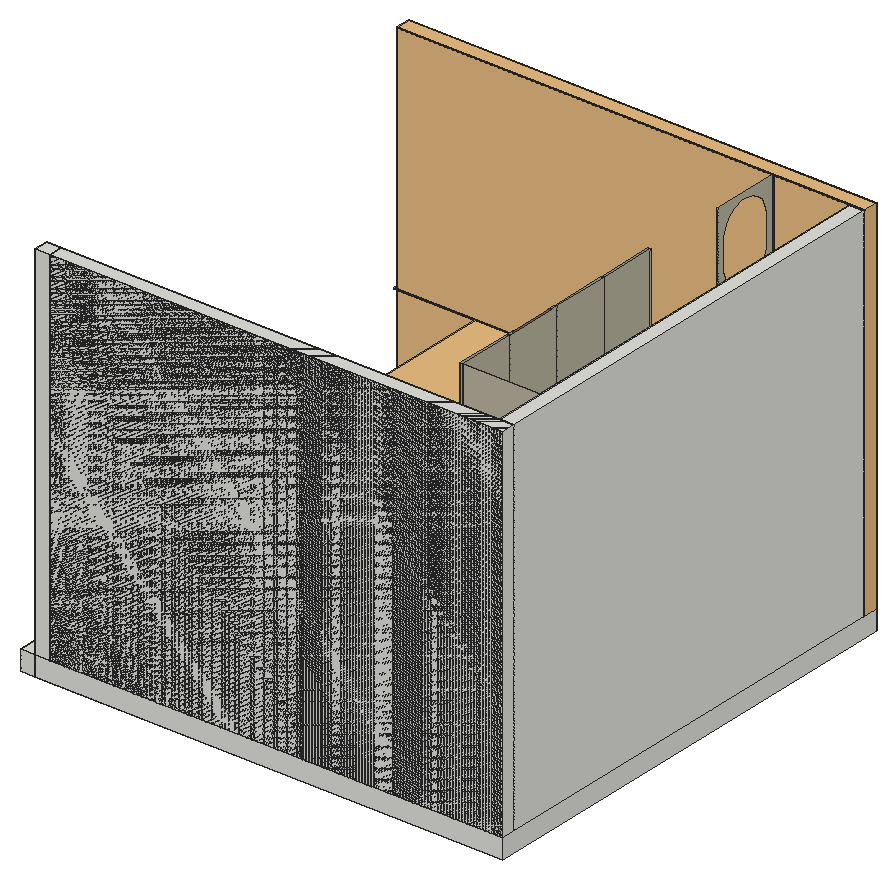
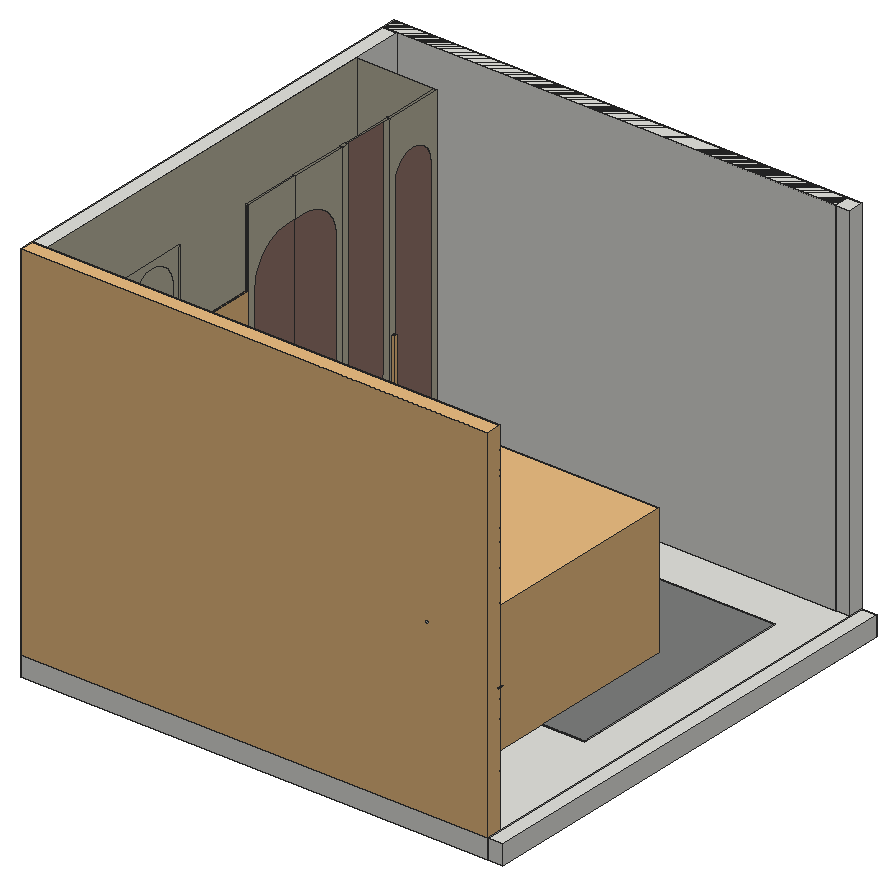
# SketchUp Ruby script. Lengths in inches.
U = 1.inch
M = Sketchup.active_model
def pt(a) = Geom::Point3d.new(a.map { |v| v * U })
def face(e, loops, mat)
  f = e.add_face(loops[0].map { |a| pt(a) })
  loops[1..].each { |l| e.add_face(l.map { |a| pt(a) }).erase! }
  f.material = f.back_material = mat if mat
  f
end
# faces: each face lists its corners as indices into pts; further lists are holes
def faces(e, pts, list, mat = nil) = list.each { |f| face(e, (f[0].is_a?(Array) ? f : [f]).map { |l| l.map { |i| pts[i] } }, mat) }
# xy, xz, yz: faces in a plane at the given z, y or x. An outline is a flat list of corners, or four numbers for a rectangle; further outlines are holes
def ring(l) = l.size == 4 ? [[l[0], l[1]], [l[2], l[1]], [l[2], l[3]], [l[0], l[3]]] : l.each_slice(2).to_a
def flat(e, list, mat, &to3) = list.each { |f| face(e, (f[0].is_a?(Array) ? f : [f]).map { |l| ring(l).map { |u, v| to3.(u, v) } }, mat) }
def xy(e, z, list, mat = nil) = flat(e, list, mat) { |x, y| [x, y, z] }
def xz(e, y, list, mat = nil) = flat(e, list, mat) { |x, z| [x, y, z] }
def yz(e, x, list, mat = nil) = flat(e, list, mat) { |y, z| [x, y, z] }
def lines(e, pts, list) = list.each { |a, b| e.add_line(pt(pts[a]), pt(pts[b])) }
# prism: a flat outline (further loops are holes) pulled along v
def prism(e, loops, v, mat = nil)
  f = face(e, loops, mat); d = Geom::Vector3d.new(v.map { |x| x * U })
  f.pushpull(f.normal.samedirection?(d) ? d.length : -d.length)
end
def box(e, o, s, mat = nil) = prism(e, [[o, [o[0] + s[0], o[1], o[2]], [o[0] + s[0], o[1] + s[1], o[2]], [o[0], o[1] + s[1], o[2]]]], [0, 0, s[2]], mat)
def at(x, y, z, deg = 0) = Geom::Transformation.translation(pt([x, y, z])) * Geom::Transformation.rotation(ORIGIN, Z_AXIS, deg.degrees)
def axes(o, x, y, z) = Geom::Transformation.new([*x, 0, *y, 0, *z, 0, *pt(o).to_a, 1])
def part(name) = M.definitions.add(name)
# library, detail: a bought-in or finely detailed component or shape, given as its bounding box
def library(name, o, s) = part(name).tap { |d| box(d.entities, o, s) }
def detail(e, o, s) = box(e.add_group.entities, o, s)
def put(e, d, t, mat = nil) = e.add_instance(d, t).tap { |i| i.material = mat if mat }
def group(e, t, mat = nil) = e.add_group.tap { |g| g.transformation = t; g.material = mat if mat }.entities
root = M.entities
M.materials.add("DDR840RVS01100X").color = [126, 127, 125]
M.materials.add("Olon-Blank-Canvas-VF300-1K").color = [237, 238, 234]
M.materials.add("Tafisa-Terrarossa-PM780-4K").color = [148, 117, 107]
M.materials.add("Uniboard-L19-Putty-4K").color = [187, 181, 160]
c1 = library("Group\#10",[-0.5,-0.5,-0.1],[116.2,1.51,0.2])
c2 = library("Group149\#1",[-72,-56,0],[144,112,0.24])
c3 = part("Carpet v15 (4)")
xy(c3.entities,0,[[-70.87,0,47.24,78.74]])
xy(c3.entities,0.39,[[-70.87,0,47.24,78.74]],"DDR840RVS01100X")
xz(c3.entities,0,[[-70.87,0,47.24,0.39]])
xz(c3.entities,78.74,[[-70.87,0,47.24,0.39]])
yz(c3.entities,-70.87,[[0,0,78.74,0.39]])
yz(c3.entities,47.24,[[0,0,78.74,0.39]])
c4 = library("Crowd Pleaser Bed",[-34.48,-45.67,0],[68.96,91.51,40.05])
c5 = library("Group39\#2",[-12.88,-41.94,0],[25.76,83.88,0.5])
c6 = library("Block 237 020",[-7.27,-8.35,0],[14.55,16.7,1.34])
c7 = part("Component\#11")
detail(c7.entities,[0,0,0],[0.1875,0.74,16.72])
c8 = library("Group\#26",[-0.5,-0.5,0],[2,18,8.5])
c9 = library("Cabinet knob",[0,0,0],[1.34,1.34,0.92])
c10 = library("Group\#23",[-0.5,-0.5,-0.1],[2,18,0.2])
c11 = library("Interior Props 221 030",[-2.57,-3.63,-0.04],[5.13,7.27,11.89])
c12 = library("Group\#24",[-0.5,-0.5,0],[2,18,8.5])
c13 = library("Candle 296 011",[-2.88,-2.88,-0.03],[5.76,5.76,9.25])
c14 = library("Group\#22",[-0.5,-0.5,-0.1],[2,18,0.2])
c15 = library("Interior Props 221 025",[-7.35,-1.5,-10.4],[14.7,1.56,20.81])
c16 = library("Group\#21",[-0.5,-0.5,-0.1],[2,18,0.2])
c17 = library("Decorative Deer 209 004",[-1.58,-4.16,0],[3.36,7.25,10.63])
xy(root,6,[[122,20.22,144,139.5]],"Uniboard-L19-Putty-4K")
xy(root,10,[[119.29,56.62,119.29,58.62,119.53,58.62,119.53,74.5,120,74.5,120,56.62],[119.53,74.62,119.53,90.5,119.29,90.5,119.29,92.5,120,92.5,120,74.62]],"Tafisa-Terrarossa-PM780-4K")
xy(root,10,[[119.29,20.22,119.29,22.22,119.53,22.22,119.53,36.36,119.29,36.36,119.29,38.24,120,38.24,120,20.22],[120,20.22,122,51.5],[119.29,38.36,120,51.5],[119.29,51.5,120,56.5],[120,51.5,120,92.5,122,87.5,122,51.5],
  [122,87.5,120,92.5,120,118.5,122,123.5],[119.96,92.62,120,118.38],[120,118.5,120,139.38,120.71,139.38,120.71,139.5,122,139.5,122,123.5]],"Uniboard-L19-Putty-4K")
xy(root,17.69,[[119.29,38.36,120,56.5]],"Uniboard-L19-Putty-4K")
xy(root,17.8125,[[119.29,38.36,120,56.5]],"Uniboard-L19-Putty-4K")
xy(root,23.65,[[120,120.5,141.83,137.5]],"Uniboard-L19-Putty-4K")
xy(root,24.35,[[120,120.5,142.83,137.5]],"Uniboard-L19-Putty-4K")
xy(root,25.51,[[119.29,38.36,120,56.5]],"Uniboard-L19-Putty-4K")
xy(root,25.625,[[119.29,38.36,120,56.5]],"Uniboard-L19-Putty-4K")
xy(root,33.32,[[119.29,38.36,120,56.5]],"Uniboard-L19-Putty-4K")
xy(root,33.4375,[[119.29,38.36,120,56.5]],"Uniboard-L19-Putty-4K")
xy(root,41.13,[[119.29,38.36,120,56.5]],"Uniboard-L19-Putty-4K")
xy(root,41.25,[[119.29,38.36,120,56.5]],"Uniboard-L19-Putty-4K")
xy(root,46.5,[[120,120.5,141.83,137.5]],"Uniboard-L19-Putty-4K")
xy(root,47.21,[[120,120.5,142.83,137.5]],"Uniboard-L19-Putty-4K")
xy(root,63.29,[[120,120.5,141.83,137.5]],"Uniboard-L19-Putty-4K")
xy(root,64,[[120,120.5,142.83,137.5]],"Uniboard-L19-Putty-4K")
xz(root,20.22,[[122,6,144,6,144,118,120,118,120,10,122,10],[119.29,10,120,117.88]],"Uniboard-L19-Putty-4K")
xz(root,22.22,[[119.29,10,119.53,99.06]],"Tafisa-Terrarossa-PM780-4K")
xz(root,36.36,[[119.29,10,119.53,99.06]],"Tafisa-Terrarossa-PM780-4K")
xz(root,38.24,[[119.29,10,120,117.88]],"Uniboard-L19-Putty-4K")
xz(root,38.36,[[119.29,10,120,17.69],[119.29,17.8125,120,25.51],[119.29,25.51,120,25.625],[119.29,25.625,120,33.32],[119.29,33.4375,120,41.13],
  [119.29,41.25,120,117.88]],"Uniboard-L19-Putty-4K")
xz(root,40.36,[[119.29,50.32,119.53,117.88]],"Tafisa-Terrarossa-PM780-4K")
xz(root,54.5,[[119.29,50.32,119.53,117.88]],"Tafisa-Terrarossa-PM780-4K")
xz(root,56.5,[[119.29,10,120,17.69],[119.29,17.8125,120,25.51],[119.29,25.625,120,33.32],[119.29,33.4375,120,41.13],[119.29,41.25,119.29,117.88,119.53,117.88,119.53,118,120,118,120,41.25]],"Uniboard-L19-Putty-4K")
xz(root,56.62,[[119.29,10,120,117.88]],"Uniboard-L19-Putty-4K")
xz(root,58.62,[[119.29,10,119.53,94.14]],"Tafisa-Terrarossa-PM780-4K")
xz(root,74.5,[[119.53,10,119.53,106.125,119.29,106.125,119.29,117.88,120,117.88,120,10]],"Tafisa-Terrarossa-PM780-4K")
xz(root,74.62,[[119.53,10,120,10,120,117.88,119.29,117.88,119.29,106.125,119.53,106.125]],"Tafisa-Terrarossa-PM780-4K")
xz(root,90.5,[[119.29,10,119.53,93.8125]],"Tafisa-Terrarossa-PM780-4K")
xz(root,92.5,[[119.29,10,120,117.88]],"Uniboard-L19-Putty-4K")
xz(root,92.62,[[119.96,10,120,93.88]],"Uniboard-L19-Putty-4K")
xz(root,118.38,[[119.96,10,120,93.88]],"Uniboard-L19-Putty-4K")
xz(root,120.5,[[120,20.5,142.83,23.65],[120,24.35,142.83,27.5],[120,47.21,142.83,63.29],[120,64,142.83,80.79]],"Uniboard-L19-Putty-4K")
xz(root,137.5,[[120,20.5,142.83,23.65],[120,24.35,142.83,27.5],[120,47.21,142.83,63.29],[120,64,142.83,80.79]],"Uniboard-L19-Putty-4K")
xz(root,139.38,[[120,10,120.71,117.88]],"Uniboard-L19-Putty-4K")
xz(root,139.5,[[122,6,122,10,120.71,10,120.71,118,144,118,144,6]],"Uniboard-L19-Putty-4K")
xz(root,146.875,[[20.87,60.82,20.98,61.01,21.19,61.01,21.09,61.19,21.19,61.38,20.98,61.38,20.87,61.57,20.76,61.38,20.54,61.38,20.65,61.19,20.76,61.01],[20.54,61.01,20.76,61.01,20.65,61.19]])
yz(root,119.29,[[20.22,10,20.22,117.88,38.24,117.88,38.24,10,36.36,10,36.36,99.06,36.3,99.98,36.12,100.89,35.82,101.76,35.41,102.59,34.9,103.36,34.29,104.05,33.6,104.66,32.83,105.18,32,105.59,31.12,105.88,30.22,106.06,29.29,106.125,28.37,106.06,27.46,105.88,26.59,105.59,25.76,105.18,24.99,104.66,24.29,104.05,23.68,103.36,23.17,102.59,22.76,101.76,22.46,100.89,22.28,99.98,22.22,99.06,22.22,10],[38.36,10,56.5,17.69],[56.62,10,56.62,117.88,74.5,117.88,74.5,106.125,70.41,106.125,70.22,106.12,70.04,106.11,69.66,106.09,69.47,106.07,69.29,106.05,68.91,106.01,68.73,105.98,68.54,105.95,68.35,105.91,67.99,105.84,67.8,105.79,67.62,105.75,67.4375,105.7,67.26,105.65,67.08,105.6,66.54,105.42,66.36,105.35,66.1875,105.28,66.01,105.21,65.84,105.14,65.67,105.0625,65.5,104.98,65.16,104.82,64.99,104.73,64.83,104.64,64.66,104.55,64.5,104.46,64.02,104.16,63.87,104.05,63.71,103.95,63.56,103.84,63.41,103.72,63.26,103.61,63.11,103.49,62.96,103.375,62.82,103.25,62.54,103.01,62.26,102.75,62.13,102.62,62,102.48,61.87,102.35,61.61,102.07,61.49,101.92,61.37,101.78,61.25,101.63,61.13,101.49,61.02,101.34,60.91,101.1875,60.8,101.03,60.69,100.88,60.59,100.72,60.48,100.5625,60.38,100.4,60.29,100.24,60.19,100.08,60.1,99.92,59.92,99.58,59.6,98.9,59.53,98.73,59.46,98.55,59.39,98.38,59.33,98.2,59.26,98.02,59.2,97.85,59.15,97.67,59.09,97.49,59.04,97.3,58.99,97.12,58.91,96.76,58.87,96.57,58.83,96.39,58.8,96.2,58.77,96.02,58.71,95.64,58.69,95.46,58.67,95.27,58.66,95.08,58.64,94.9,58.63,94.71,58.62,94.33,58.62,10],[90.5,10,90.5,93.8125,90.39,95.42,90.08,97,89.5625,98.52,88.85,99.97,87.96,101.31,86.89,102.52,85.68,103.58,84.34,104.48,82.9,105.1875,81.375,105.71,79.79,106.02,78.1875,106.125,74.62,106.125,74.62,117.88,92.5,117.88,92.5,10],[38.24,17.8125,38.36,25.625],
  [38.36,17.8125,56.5,25.51],[38.36,25.625,56.5,33.32],[38.36,33.4375,56.5,41.13],[38.36,41.25,38.36,117.88,40.36,117.88,40.36,50.32,40.42,49.4,40.6,48.49,40.9,47.61,41.31,46.78,41.82,46.02,42.43,45.32,43.13,44.71,43.9,44.2,44.73,43.79,45.6,43.49,46.51,43.31,47.43,43.25,48.35,43.31,49.26,43.49,50.14,43.79,50.97,44.2,51.73,44.71,52.43,45.32,53.04,46.02,53.55,46.78,53.96,47.61,54.26,48.49,54.44,49.4,54.5,50.32,54.5,117.88,56.5,117.88,56.5,41.25]],"Uniboard-L19-Putty-4K")
yz(root,119.53,[[22.22,10,22.22,99.06,22.28,99.98,22.46,100.89,22.76,101.76,23.17,102.59,23.68,103.36,24.29,104.05,24.99,104.66,25.76,105.18,26.59,105.59,27.46,105.88,28.37,106.06,29.29,106.125,30.22,106.06,31.12,105.88,32,105.59,32.83,105.18,33.6,104.66,34.29,104.05,34.9,103.36,35.41,102.59,35.82,101.76,36.12,100.89,36.3,99.98,36.36,99.06,36.36,10],[58.62,10,58.62,94.33,58.63,94.71,58.64,94.9,58.66,95.08,58.67,95.27,58.69,95.46,58.71,95.64,58.77,96.02,58.8,96.2,58.83,96.39,58.87,96.57,58.91,96.76,58.99,97.12,59.04,97.3,59.09,97.49,59.15,97.67,59.2,97.85,59.26,98.02,59.33,98.2,59.39,98.38,59.46,98.55,59.53,98.73,59.6,98.9,59.92,99.58,60.1,99.92,60.19,100.08,60.29,100.24,60.38,100.4,60.48,100.5625,60.59,100.72,60.69,100.88,60.8,101.03,60.91,101.1875,61.02,101.34,61.13,101.49,61.25,101.63,61.37,101.78,61.49,101.92,61.61,102.07,61.87,102.35,62,102.48,62.13,102.62,62.26,102.75,62.54,103.01,62.82,103.25,62.96,103.375,63.11,103.49,63.26,103.61,63.41,103.72,63.56,103.84,63.71,103.95,63.87,104.05,64.02,104.16,64.5,104.46,64.66,104.55,64.83,104.64,64.99,104.73,65.16,104.82,65.5,104.98,65.67,105.0625,65.84,105.14,66.01,105.21,66.1875,105.28,66.36,105.35,66.54,105.42,67.08,105.6,67.26,105.65,67.4375,105.7,67.62,105.75,67.8,105.79,67.99,105.84,68.35,105.91,68.54,105.95,68.73,105.98,68.91,106.01,69.29,106.05,69.47,106.07,69.66,106.09,70.04,106.11,70.22,106.12,70.41,106.125,74.5,106.125,74.5,10],[74.62,10,74.62,106.125,78.1875,106.125,79.79,106.02,81.375,105.71,82.9,105.1875,84.34,104.48,85.68,103.58,86.89,102.52,87.96,101.31,88.85,99.97,89.5625,98.52,90.08,97,90.39,95.42,90.5,93.8125,90.5,10],[47.43,43.25,46.51,43.31,45.6,43.49,44.73,43.79,43.9,44.2,43.13,44.71,42.43,45.32,41.82,46.02,41.31,46.78,40.9,47.61,40.6,48.49,40.42,49.4,40.36,50.32,40.36,117.88,54.5,117.88,54.5,50.32,54.44,49.4,54.26,48.49,53.96,47.61,53.55,46.78,53.04,46.02,52.43,45.32,51.73,44.71,50.97,44.2,50.14,43.79,49.26,43.49,48.35,43.31]],"Tafisa-Terrarossa-PM780-4K")
yz(root,120,[[20.22,10,38.24,117.88],[38.24,10,38.36,118],[38.36,10,56.5,17.69],[56.5,10,56.62,118],[56.62,10,74.5,117.88],
  [74.5,10,74.62,118],[74.62,10,92.5,117.88],[92.5,10,92.62,118],[92.62,10,118.38,93.88],[118.38,10,118.5,118],
  [[118.5,10,139.38,117.88],[129,38,130.11,38.07,131.2,38.29,132.25,38.65,133.25,39.14,134.17,39.76,135.01,40.49,135.74,41.33,136.36,42.25,136.85,43.25,137.21,44.3,137.43,45.39,137.5,46.5,137.5,81.5,137.43,82.61,137.21,83.7,136.85,84.75,136.36,85.75,135.74,86.67,135.01,87.51,134.17,88.24,133.25,88.86,132.25,89.35,131.2,89.71,130.11,89.93,129,90,127.89,89.93,126.8,89.71,125.75,89.35,124.75,88.86,123.83,88.24,122.99,87.51,122.26,86.67,121.64,85.75,121.15,84.75,120.79,83.7,120.57,82.61,120.5,81.5,120.5,46.5,120.57,45.39,120.79,44.3,121.15,43.25,121.64,42.25,122.26,41.33,122.99,40.49,123.83,39.76,124.75,39.14,125.75,38.65,126.8,38.29,127.89,38.07],[129,92,130.05,92.06,131.08,92.26,132.08,92.58,133.04,93.02,133.93,93.57,134.75,94.23,135.48,94.98,136.12,95.82,136.64,96.73,137.05,97.7,137.34,98.71,137.5,99.75,137.5,107.5,137.43,108.61,137.21,109.7,136.85,110.75,136.36,111.75,135.74,112.67,135.01,113.51,134.17,114.24,133.25,114.86,132.25,115.35,131.2,115.71,130.11,115.93,129,116,127.89,115.93,126.8,115.71,125.75,115.35,124.75,114.86,123.83,114.24,122.99,113.51,122.26,112.67,121.64,111.75,121.15,110.75,120.79,109.7,120.57,108.61,120.5,107.5,120.5,100.5,120.57,99.39,120.79,98.3,121.15,97.25,121.64,96.25,122.26,95.33,122.99,94.49,123.83,93.76,124.75,93.14,125.75,92.65,126.8,92.29,127.89,92.07],[129,12,130.11,12.07,131.2,12.29,132.25,12.65,133.25,13.14,134.17,13.76,135.01,14.49,135.74,15.33,136.36,16.25,136.85,17.25,137.21,18.3,137.43,19.39,137.5,20.5,137.5,27.5,137.43,28.61,137.21,29.7,136.85,30.75,136.36,31.75,135.74,32.67,135.01,33.51,134.17,34.24,133.25,34.86,132.25,35.35,131.2,35.71,130.11,35.93,129,36,127.89,35.93,126.8,35.71,125.75,35.35,124.75,34.86,123.83,34.24,122.99,33.51,122.26,32.67,121.64,31.75,121.15,30.75,120.79,29.7,120.57,28.61,120.5,27.5,120.5,20.5,120.57,19.39,120.79,18.3,121.15,17.25,121.64,16.25,122.26,15.33,122.99,14.49,123.83,13.76,124.75,13.14,125.75,12.65,126.8,12.29,127.89,12.07]],[38.36,17.69,56.5,17.8125],[38.36,17.8125,56.5,25.51],[120.5,23.65,137.5,24.35],[38.36,25.51,56.5,25.625],
  [38.36,25.625,56.5,33.32],[38.36,33.32,56.5,33.4375],[38.36,33.4375,56.5,41.13],[38.36,41.13,56.5,41.25],[38.36,41.25,56.5,41.25,56.5,118,54.5,118,54.5,117.88,38.36,117.88],
  [120.5,46.5,137.5,47.21],[120.5,63.29,137.5,64]],"Uniboard-L19-Putty-4K")
yz(root,120.71,[[139.38,10,139.5,118]],"Uniboard-L19-Putty-4K")
yz(root,122,[[20.22,6,51.5,10],[51.5,6,139.5,10]],"Uniboard-L19-Putty-4K")
yz(root,142.83,[[129,12,127.89,12.07,126.8,12.29,125.75,12.65,124.75,13.14,123.83,13.76,122.99,14.49,122.26,15.33,121.64,16.25,121.15,17.25,120.79,18.3,120.57,19.39,120.5,20.5,120.5,23.65,137.5,23.65,137.5,20.5,137.43,19.39,137.21,18.3,136.85,17.25,136.36,16.25,135.74,15.33,135.01,14.49,134.17,13.76,133.25,13.14,132.25,12.65,131.2,12.29,130.11,12.07],[120.5,24.35,120.5,27.5,120.57,28.61,120.79,29.7,121.15,30.75,121.64,31.75,122.26,32.67,122.99,33.51,123.83,34.24,124.75,34.86,125.75,35.35,126.8,35.71,127.89,35.93,129,36,130.11,35.93,131.2,35.71,132.25,35.35,133.25,34.86,134.17,34.24,135.01,33.51,135.74,32.67,136.36,31.75,136.85,30.75,137.21,29.7,137.43,28.61,137.5,27.5,137.5,24.35],[129,38,127.89,38.07,126.8,38.29,125.75,38.65,124.75,39.14,123.83,39.76,122.99,40.49,122.26,41.33,121.64,42.25,121.15,43.25,120.79,44.3,120.57,45.39,120.5,46.5,137.5,46.5,137.43,45.39,137.21,44.3,136.85,43.25,136.36,42.25,135.74,41.33,135.01,40.49,134.17,39.76,133.25,39.14,132.25,38.65,131.2,38.29,130.11,38.07],[120.5,47.21,137.5,63.29],[120.5,64,137.5,80.79]],"Uniboard-L19-Putty-4K")
yz(root,144,[[20.22,6,139.5,118]],"Uniboard-L19-Putty-4K")
p = [[120,127.89,12.07],[141.83,127.89,12.07],[141.83,129,12],[120,129,12],[141.83,130.11,12.07],[120,130.11,12.07],
  [120,126.8,12.29],[141.83,126.8,12.29],[141.83,131.2,12.29],[120,131.2,12.29],[120,125.75,12.65],[141.83,125.75,12.65],
  [141.83,132.25,12.65],[120,132.25,12.65],[120,124.75,13.14],[141.83,124.75,13.14],[141.83,133.25,13.14],[120,133.25,13.14],
  [120,123.83,13.76],[141.83,123.83,13.76],[141.83,134.17,13.76],[120,134.17,13.76],[120,122.99,14.49],[141.83,122.99,14.49],
  [141.83,135.01,14.49],[120,135.01,14.49],[120,122.26,15.33],[141.83,122.26,15.33],[141.83,135.74,15.33],[120,135.74,15.33],
  [120,121.64,16.25],[141.83,121.64,16.25],[141.83,136.36,16.25],[120,136.36,16.25],[120,121.15,17.25],[141.83,121.15,17.25],
  [141.83,136.85,17.25],[120,136.85,17.25],[120,120.79,18.3],[141.83,120.79,18.3],[141.83,137.21,18.3],[120,137.21,18.3],
  [120,120.57,19.39],[141.83,120.57,19.39],[141.83,137.43,19.39],[120,137.43,19.39],[120,120.5,20.5],[141.83,120.5,20.5],
  [141.83,137.5,20.5],[120,137.5,20.5],[120,120.57,28.61],[141.83,120.57,28.61],[141.83,120.5,27.5],[120,120.5,27.5],
  [120,137.5,27.5],[141.83,137.5,27.5],[141.83,137.43,28.61],[120,137.43,28.61],[120,120.79,29.7],[141.83,120.79,29.7],
  [141.83,137.21,29.7],[120,137.21,29.7],[120,121.15,30.75],[141.83,121.15,30.75],[141.83,136.85,30.75],[120,136.85,30.75],
  [120,121.64,31.75],[141.83,121.64,31.75],[141.83,136.36,31.75],[120,136.36,31.75],[120,122.26,32.67],[141.83,122.26,32.67],
  [141.83,135.74,32.67],[120,135.74,32.67],[120,122.99,33.51],[141.83,122.99,33.51],[141.83,135.01,33.51],[120,135.01,33.51],
  [120,123.83,34.24],[141.83,123.83,34.24],[141.83,134.17,34.24],[120,134.17,34.24],[120,124.75,34.86],[141.83,124.75,34.86],
  [141.83,133.25,34.86],[120,133.25,34.86],[120,125.75,35.35],[141.83,125.75,35.35],[141.83,132.25,35.35],[120,132.25,35.35],
  [120,126.8,35.71],[141.83,126.8,35.71],[141.83,131.2,35.71],[120,131.2,35.71],[120,127.89,35.93],[141.83,127.89,35.93],
  [141.83,130.11,35.93],[120,130.11,35.93],[120,129,36],[141.83,129,36],[120,129,38],[120,127.89,38.07],
  [142.83,127.89,38.07],[142.83,129,38],[120,130.11,38.07],[142.83,130.11,38.07],[120,126.8,38.29],[142.83,126.8,38.29],
  [120,131.2,38.29],[142.83,131.2,38.29],[120,125.75,38.65],[142.83,125.75,38.65],[120,132.25,38.65],[142.83,132.25,38.65],
  [120,124.75,39.14],[142.83,124.75,39.14],[120,133.25,39.14],[142.83,133.25,39.14],[120,123.83,39.76],[142.83,123.83,39.76],
  [120,134.17,39.76],[142.83,134.17,39.76],[120,122.99,40.49],[142.83,122.99,40.49],[120,135.01,40.49],[142.83,135.01,40.49],
  [120,122.26,41.33],[142.83,122.26,41.33],[120,135.74,41.33],[142.83,135.74,41.33],[120,121.64,42.25],[142.83,121.64,42.25],
  [120,136.36,42.25],[142.83,136.36,42.25],[120,121.15,43.25],[142.83,121.15,43.25],[120,136.85,43.25],[142.83,136.85,43.25],
  [119.29,47.43,43.25],[119.29,46.51,43.31],[119.53,46.51,43.31],[119.53,47.43,43.25],[119.29,48.35,43.31],[119.53,48.35,43.31],
  [120,120.79,44.3],[142.83,120.79,44.3],[120,137.21,44.3],[142.83,137.21,44.3],[119.29,45.6,43.49],[119.53,45.6,43.49],
  [119.29,49.26,43.49],[119.53,49.26,43.49],[119.29,44.73,43.79],[119.53,44.73,43.79],[119.29,50.14,43.79],[119.53,50.14,43.79],
  [119.29,43.9,44.2],[119.53,43.9,44.2],[119.29,50.97,44.2],[119.53,50.97,44.2],[119.29,43.13,44.71],[119.53,43.13,44.71],
  [119.29,51.73,44.71],[119.53,51.73,44.71],[120,120.57,45.39],[142.83,120.57,45.39],[120,137.43,45.39],[142.83,137.43,45.39],
  [119.29,42.43,45.32],[119.53,42.43,45.32],[119.29,52.43,45.32],[119.53,52.43,45.32],[119.29,41.82,46.02],[119.53,41.82,46.02],
  [119.29,53.04,46.02],[119.53,53.04,46.02],[120,120.5,46.5],[141.83,120.5,46.5],[141.85,120.5,46.5],[142.83,120.5,46.5],
  [120,137.5,46.5],[142.83,137.5,46.5],[141.83,137.5,46.5],[119.29,41.31,46.78],[119.53,41.31,46.78],[119.29,53.55,46.78],
  [119.53,53.55,46.78],[119.29,40.9,47.61],[119.53,40.9,47.61],[119.29,53.96,47.61],[119.53,53.96,47.61],[119.29,40.6,48.49],
  [119.53,40.6,48.49],[119.29,54.26,48.49],[119.53,54.26,48.49],[119.29,40.42,49.4],[119.53,40.42,49.4],[119.29,54.44,49.4],
  [119.53,54.44,49.4],[119.29,40.36,50.32],[119.53,40.36,50.32],[119.29,54.5,50.32],[119.53,54.5,50.32],[141.85,120.33,46.5]]
faces(root,p,[[0,1,2,3],[3,2,4,5],[6,7,1,0],[5,4,8,9],[10,11,7,6],[9,8,12,13],[14,15,11,10],[13,12,16,17],
  [18,19,15,14],[17,16,20,21],[22,23,19,18],[21,20,24,25],[26,27,23,22],[25,24,28,29],[30,31,27,26],[29,28,32,33],
  [34,35,31,30],[33,32,36,37],[38,39,35,34],[37,36,40,41],[42,43,39,38],[41,40,44,45],[46,47,43,42],[45,44,48,49],
  [50,51,52,53],[54,55,56,57],[58,59,51,50],[57,56,60,61],[62,63,59,58],[61,60,64,65],[66,67,63,62],[65,64,68,69],
  [70,71,67,66],[69,68,72,73],[74,75,71,70],[73,72,76,77],[78,79,75,74],[77,76,80,81],[82,83,79,78],[81,80,84,85],
  [86,87,83,82],[85,84,88,89],[90,91,87,86],[89,88,92,93],[94,95,91,90],[93,92,96,97],[98,99,95,94],[97,96,99,98],
  [100,101,102,103],[104,100,103,105],[101,106,107,102],[108,104,105,109],[106,110,111,107],[112,108,109,113],[110,114,115,111],[116,112,113,117],
  [114,118,119,115],[120,116,117,121],[118,122,123,119],[124,120,121,125],[122,126,127,123],[128,124,125,129],[126,130,131,127],[132,128,129,133],
  [130,134,135,131],[136,132,133,137],[134,144,145,135],[146,136,137,147],[144,164,165,145],[166,146,147,167],[164,176,177,178,179,165],[180,166,167,181,182]],"Uniboard-L19-Putty-4K")
faces(root,p,[[138,139,140,141],[142,138,141,143],[139,148,149,140],[150,142,143,151],[148,152,153,149],[154,150,151,155],[152,156,157,153],[158,154,155,159],
  [156,160,161,157],[162,158,159,163],[160,168,169,161],[170,162,163,171],[168,172,173,169],[174,170,171,175],[172,183,184,173],[185,174,175,186],
  [183,187,188,184],[189,185,186,190],[187,191,192,188],[193,189,190,194],[191,195,196,192],[197,193,194,198],[195,199,200,196],[201,197,198,202]],"Tafisa-Terrarossa-PM780-4K")
lines(root,p,[[178,203]])
g1 = group(root,at(4.5,0,0))
xy(g1,0,[[-4.5,0,0,144],[0,0,144,144]])
xy(g1,6,[[-4.5,0,0,144],[0,0,144,144]])
xz(g1,0,[[-4.5,0,0,6],[0,0,144,6]])
xz(g1,144,[[-4.5,0,0,6],[0,0,144,6]])
yz(g1,-4.5,[[0,0,144,6]])
yz(g1,0,[[0,0,144,6]])
yz(g1,144,[[0,0,144,6]])
g2 = group(root,at(144,4.5,6))
box(g2,[0,0,0],[4.5,135,112])
g3 = group(root,at(9,0,6))
box(g3,[0,0,0],[139.5,4.5,112])
g4 = group(root,at(4.5,139.5,6))
xz(g4,0,[[110.0625,95.3,110.33,95.77,110.875,95.77,110.6,96.24,110.875,96.71,110.33,96.71,110.0625,97.18,109.79,96.71,109.25,96.71,109.52,96.24,109.25,95.77,109.79,95.77]],"Olon-Blank-Canvas-VF300-1K")
xz(g4,0.51,[[108.47,76.29,108.74,76.76,109.28,76.76,109.01,77.23,109.28,77.7,108.74,77.7,108.47,78.17,108.2,77.7,107.65,77.7,107.93,77.23,107.65,76.76,108.2,76.76]],"Olon-Blank-Canvas-VF300-1K")
p = [[115.2,0,40],[0,0,40],[68.98,0.75,57.76],[69.08,0.75,57.62],[69.17,0.75,57.48],[69.25,0.75,57.33],
  [69.33,0.75,57.18],[69.36,0.75,57.11],[69.4,0.75,57.03],[69.47,0.75,56.87],[69.54,0.75,56.72],[69.6,0.75,56.56],
  [69.65,0.75,56.4],[69.7,0.75,56.23],[69.75,0.75,56.07],[69.79,0.75,55.91],[69.82,0.75,55.74],[69.85,0.75,55.57],
  [69.875,0.75,55.4],[69.9,0.75,55.23],[59.16,0.75,55.5],[59.16,0.75,55.51],[88.41,0.75,59.52],[88.38,0.75,59.12],
  [88.34,0.75,58.71],[88.28,0.75,58.31],[88.2,0.75,57.91],[88.11,0.75,57.51],[88,0.75,57.11],[87.88,0.75,56.73],
  [87.74,0.75,56.34],[87.58,0.75,55.97],[87.41,0.75,55.6],[87.22,0.75,55.23],[68.92,0.75,57.85],[104.2,0.75,57.11],
  [104.25,0.75,56.84],[104.3,0.75,56.58],[104.34,0.75,56.3125],[104.37,0.75,56.04],[104.39,0.75,55.77],[104.4,0.75,55.5],
  [104.41,0.75,55.23],[88.41,0.75,59.6],[104.16,0.75,57.26],[12.07,0.75,65.78],[11.99,0.75,65.59],[11.9,0.75,65.39],
  [11.8,0.75,65.2],[50.17,0.75,54.73],[50.27,0.75,54.91],[50.36,0.75,55.1],[50.45,0.75,55.3],[50.53,0.75,55.5],
  [50.6,0.75,55.7],[50.66,0.75,55.9],[50.71,0.75,56.11],[50.75,0.75,56.32],[50.78,0.75,56.53],[50.81,0.75,56.74],
  [50.83,0.75,56.95],[50.83,0.75,57.17],[50.83,0.75,57.38],[50.82,0.75,57.59],[50.8,0.75,57.8],[50.8,0.75,57.84],
  [41.32,0.75,59.8125],[41.22,0.75,59.63],[41.12,0.75,59.4375],[41.04,0.75,59.24],[40.96,0.75,59.04],[40.88,0.75,58.84],
  [40.82,0.75,58.64],[40.77,0.75,58.43],[40.72,0.75,58.23],[40.6875,0.75,58.02],[40.66,0.75,57.8],[40.64,0.75,57.59],
  [40.63,0.75,57.38],[40.63,0.75,57.17],[40.64,0.75,56.95],[40.65,0.75,56.74],[40.68,0.75,56.53],[40.71,0.75,56.32],
  [40.76,0.75,56.11],[40.81,0.75,55.9],[40.87,0.75,55.7],[40.9375,0.75,55.5],[41.01,0.75,55.3],[41.1,0.75,55.1],
  [41.19,0.75,54.91],[41.29,0.75,54.73],[26.15,0.75,61.03],[26.03,0.75,60.77],[25.91,0.75,60.51],[25.81,0.75,60.24],
  [25.72,0.75,59.98],[25.63,0.75,59.7],[25.56,0.75,59.43],[25.49,0.75,59.15],[25.4375,0.75,58.87],[25.39,0.75,58.59],
  [25.35,0.75,58.31],[25.33,0.75,58.02],[25.3125,0.75,57.74],[25.31,0.75,57.45],[41.36,0.75,59.88],[26.2,0.75,61.14],
  [71.89,0.75,82.62],[72.01,0.75,82.53],[71.73,0.75,83.01],[71.74,0.75,82.87],[71.8,0.75,82.73],[72.14,0.75,82.47],
  [72.29,0.75,82.45],[72.43,0.75,82.47],[72.57,0.75,82.53],[72.6875,0.75,82.62],[72.78,0.75,82.73],[72.83,0.75,82.87],
  [72.85,0.75,83.01],[68.68,0.75,82.62],[68.8,0.75,82.53],[68.52,0.75,83.01],[68.53,0.75,82.94],[68.54,0.75,82.87],
  [68.59,0.75,82.73],[68.9375,0.75,82.47],[69.08,0.75,82.45],[69.23,0.75,82.47],[69.36,0.75,82.53],[69.48,0.75,82.62],
  [69.57,0.75,82.73],[69.625,0.75,82.87],[69.64,0.75,83.01],[68.54,0.75,83.01],[70.38,0.75,79.15],[70.52,0.75,79.09],
  [70.11,0.75,79.5625],[70.12,0.75,79.49],[70.18,0.75,79.35],[70.27,0.75,79.24],[70.67,0.75,79.07],[70.8125,0.75,79.09],
  [70.95,0.75,79.15],[71.0625,0.75,79.24],[71.15,0.75,79.35],[71.21,0.75,79.49],[71.23,0.75,79.63],[70.1,0.75,79.63],
  [70.12,0.75,79.63]]
lines(g4,p,[[0,1],[2,3],[3,4],[4,5],[5,6],[6,7],[8,9],[9,10],[10,11],[11,12],[12,13],[13,14],
  [14,15],[15,16],[16,17],[17,18],[18,19],[20,21],[7,8],[22,23],[23,24],[24,25],[25,26],[26,27],
  [27,28],[28,29],[29,30],[30,31],[31,32],[32,33],[34,2],[35,36],[36,37],[37,38],[38,39],[39,40],
  [40,41],[41,42],[43,22],[44,35],[45,46],[46,47],[47,48],[49,50],[50,51],[51,52],[52,53],[53,54],
  [54,55],[55,56],[56,57],[57,58],[58,59],[59,60],[60,61],[61,62],[62,63],[63,64],[64,65],[66,67],
  [67,68],[68,69],[69,70],[70,71],[71,72],[72,73],[73,74],[74,75],[75,76],[76,77],[77,78],[78,79],
  [79,80],[80,81],[81,82],[82,83],[83,84],[84,85],[85,86],[86,87],[87,88],[88,89],[89,90],[90,91],
  [92,93],[93,94],[94,95],[95,96],[96,97],[97,98],[98,99],[99,100],[100,101],[101,102],[102,103],[103,104],
  [104,105],[106,66],[107,92],[108,109],[110,111],[111,112],[112,108],[109,113],[113,114],[114,115],[115,116],[116,117],
  [117,118],[118,119],[119,120],[121,122],[123,124],[125,126],[126,121],[122,127],[127,128],[128,129],[129,130],[130,131],
  [131,132],[132,133],[133,134],[124,135],[124,125],[136,137],[138,139],[139,140],[140,141],[141,136],[137,142],[142,143],
  [143,144],[144,145],[145,146],[146,147],[147,148],[149,138],[138,150]])
detail(g4,[0,0,0],[144,4.5,112])
put(g4,c1,at(0,0,40),"Uniboard-L19-Putty-4K")
put(g4,c2,axes([72,0,56],[1,0,0],[0,0,1],[0,-1,0]),"Uniboard-L19-Putty-4K")
g5 = group(root,at(4.5,0,6))
box(g5,[0,0,0],[144,4.5,112])
g6 = group(root,at(0,0,6))
xy(g6,0,[[0,0,4.5,144]])
put(root,c3,axes([75.65,19.32,6],[0.84295,0,0],[0,0.93,0],[0,0,0.93]))
put(root,c4,at(63.52,92.99,6))
put(root,c5,axes([119.96,105.5,51.94],[0,-1,0],[0,0,1],[-1,0,0]),"Uniboard-L19-Putty-4K")
put(root,c6,axes([126.83,131.78,17.8125],[0.7,0,0],[0,-0.20264,-0.67003],[0,0.67003,-0.20264]))
put(root,c6,axes([126.83,130.32,17.8125],[0.7,0,0],[0,-0.20264,-0.67003],[0,0.67003,-0.20264]))
put(root,c7,axes([119.53,75.12,12],[0,4.59482,0],[-1.67085,0,0],[0,0,2.75092]))
put(root,c7,axes([119.53,73.17,12],[0,4.59482,0],[-1.67085,0,0],[0,0,2.75092]))
put(root,c7,axes([119.29,36.91,12],[0,4.59482,0],[-1.67085,0,0],[0,0,2.75092]))
put(root,c8,at(141.83,120.5,12),"Uniboard-L19-Putty-4K")
put(root,c6,axes([126.22,128.49,17.89],[0.7,0,0],[0,-0.20264,-0.67003],[0,0.67003,-0.20264]))
put(root,c9,axes([119.29,46.72,13.4],[0,0,1],[0,1,0],[-1,0,0]),"Uniboard-L19-Putty-4K")
put(root,c9,axes([119.29,46.72,20.78],[0,0,1],[0,1,0],[-1,0,0]),"Uniboard-L19-Putty-4K")
put(root,c10,at(141.83,120.5,23.65),"Uniboard-L19-Putty-4K")
put(root,c11,axes([126.47,129.43,24.35],[0.34857,-0.93728,0],[0.93728,0.34857,0],[0,0,0.89]))
put(root,c12,at(141.83,120.5,27.5),"Uniboard-L19-Putty-4K")
put(root,c9,axes([119.29,46.72,28.59],[0,0,1],[0,1,0],[-1,0,0]),"Uniboard-L19-Putty-4K")
put(root,c9,axes([119.29,46.72,36.4],[0,0,1],[0,1,0],[-1,0,0]),"Uniboard-L19-Putty-4K")
put(root,c13,axes([124.99,129.01,38.25],[0.77,0,0],[0,0.77,0],[0,0,0.77]))
put(root,c14,at(141.83,120.5,46.5),"Uniboard-L19-Putty-4K")
put(root,c15,axes([125.52,127.54,55.07],[0.64952,-0.375,0],[0.5,0.86603,0],[0,0,0.75573]))
put(root,c15,axes([125.52,132.54,55.07],[0.64952,-0.375,0],[0.5,0.86603,0],[0,0,0.75573]))
put(root,c16,at(141.83,120.5,63.29),"Uniboard-L19-Putty-4K")
put(root,c17,axes([127.15,130.29,63.88],[0.6048,-1.2737,0],[1.2737,0.6048,0],[0,0,1.41]))
